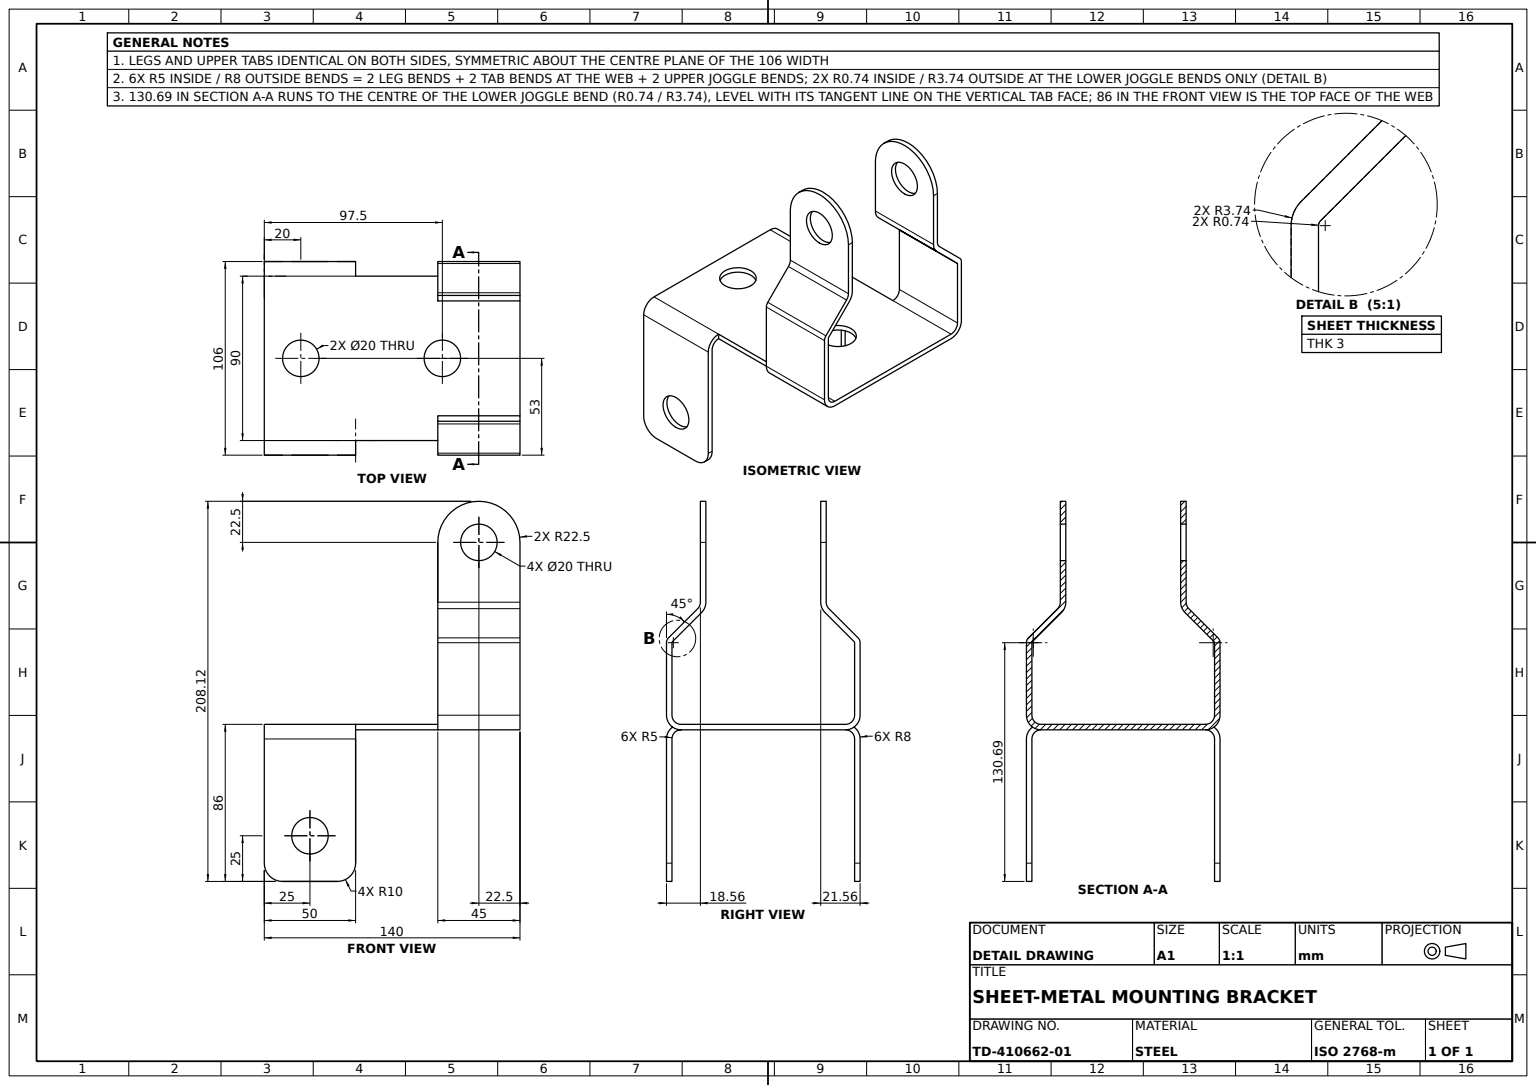
solid
v1 (-53,-76,70)
v2 (-50,-76,70)
e1 v1 v2 LINE
v3 (-50,-8,70)
e2 v2 v3 LINE
v4 (-53,-8,70)
e3 v3 v4 LINE
e4 v1 v4 LINE
face PLANE(AX(P(-53,-3,70),D(0,0,-1),D(-1,0,0))) rev [e1 e2 e3 -e4]
v5 (0,0,-17.5)
v6 (0,0,-37.5)
e5 v5 v6 CIRCLE(AX(P(0,0,-27.5),D(0,1,0),D(0,0,1)),10)
e6 v6 v5 CIRCLE(AX(P(0,0,-27.5),D(0,1,0),D(0,0,1)),10)
v7 (0,0,60)
v8 (0,0,40)
e7 v7 v8 CIRCLE(AX(P(0,0,50),D(0,1,0),D(0,0,1)),10)
e8 v8 v7 CIRCLE(AX(P(0,0,50),D(0,1,0),D(0,0,1)),10)
v9 (-45,0,-70)
v10 (-45,0,-25)
e9 v9 v10 LINE
v11 (-45,0,20)
e10 v10 v11 LINE
v12 (-45,0,70)
e11 v11 v12 LINE
v13 (45,0,70)
e12 v12 v13 LINE
v14 (45,0,20)
e13 v13 v14 LINE
v15 (45,0,-25)
e14 v14 v15 LINE
v16 (45,0,-70)
e15 v16 v15 LINE
e16 v16 v9 LINE
face PLANE(AX(P(0,0,0),D(0,-1,0),D(0,0,-1))) rev [-e5 -e6] [-e7 -e8] [e9 e10 e11 e12 e13 e14 -e15 e16]
v17 (31.443651,99.61899,-70)
v18 (31.443651,66.870058,-70)
e17 v17 v18 LINE
v19 (34.443651,99.61899,-70)
e18 v17 v19 LINE
v20 (34.443651,66.870058,-70)
e19 v19 v20 LINE
e20 v20 v18 LINE
face PLANE(AX(P(31.443651,64.79899,-70),D(0,0,1),D(1,0,0))) rev [-e17 e18 e19 e20]
v21 (50,5,-25)
e21 v15 v21 CIRCLE(AX(P(45,5,-25),D(0,0,1),D(0,1,0)),5)
v22 (50,5,-70)
e22 v21 v22 LINE
e23 v22 v16 CIRCLE(AX(P(45,5,-70),D(0,0,-1),D(0,1,0)),5)
face CYL(AX(P(45,5,-70),D(0,0,-1),D(1,0,0)),5) rev [e21 e22 e23 e15]
v23 (50,44.69489,-70)
v24 (53,44.69489,-70)
e24 v23 v24 LINE
v25 (49.784255,45.215745,-70)
e25 v25 v23 CIRCLE(AX(P(49.2634,44.69489,-70),D(0,0,-1),D(-1,0,0)),0.7366)
v26 (51.905575,47.337065,-70)
e26 v25 v26 LINE
e27 v26 v24 CIRCLE(AX(P(49.2634,44.69489,-70),D(0,0,-1),D(-1,0,0)),3.7366)
face PLANE(AX(P(49.2634,44.69489,-70),D(0,0,1),D(1,0,0))) rev [-e24 -e25 e26 e27]
v27 (-53,44.69489,-70)
v28 (-51.905575,47.337065,-70)
e28 v27 v28 CIRCLE(AX(P(-49.2634,44.69489,-70),D(0,0,-1),D(1,0,0)),3.7366)
v29 (-49.784255,45.215745,-70)
e29 v29 v28 LINE
v30 (-50,44.69489,-70)
e30 v30 v29 CIRCLE(AX(P(-49.2634,44.69489,-70),D(0,0,-1),D(1,0,0)),0.7366)
e31 v30 v27 LINE
face PLANE(AX(P(-49.2634,44.69489,-70),D(0,0,-1),D(-1,0,0))) [e28 -e29 -e30 e31]
v31 (-53,-8,20)
e32 v31 v4 LINE
v32 (-53,-76,20)
e33 v31 v32 LINE
v33 (-53,-86,30)
e34 v32 v33 CIRCLE(AX(P(-53,-76,30),D(-1,0,0),D(0,1,0)),10)
v34 (-53,-86,60)
e35 v33 v34 LINE
e36 v34 v1 CIRCLE(AX(P(-53,-76,60),D(-1,0,0),D(0,1,0)),10)
v35 (-53,-71,45)
v36 (-53,-51,45)
e37 v35 v36 CIRCLE(AX(P(-53,-61,45),D(-1,0,0),D(0,-1,0)),10)
e38 v36 v35 CIRCLE(AX(P(-53,-61,45),D(-1,0,0),D(0,-1,0)),10)
face PLANE(AX(P(-53,0,0),D(1,0,0),D(0,1,0))) rev [-e32 e33 e34 e35 e36 e4] [-e37 -e38]
v37 (-34.443651,66.870058,-25)
v38 (-31.443651,66.870058,-25)
e39 v37 v38 LINE
v39 (-35.908117,63.334524,-25)
e40 v39 v37 CIRCLE(AX(P(-39.443651,66.870058,-25),D(0,0,1),D(-1,0,0)),5)
v40 (-33.786797,61.213203,-25)
e41 v39 v40 LINE
e42 v40 v38 CIRCLE(AX(P(-39.443651,66.870058,-25),D(0,0,1),D(-1,0,0)),8)
face PLANE(AX(P(-39.443651,66.870058,-25),D(0,0,1),D(1,0,0))) [-e39 -e40 e41 e42]
v41 (-51.905575,47.337065,-25)
v42 (-53,44.69489,-25)
e43 v41 v42 CIRCLE(AX(P(-49.2634,44.69489,-25),D(0,0,1),D(1,0,0)),3.7366)
v43 (-50,44.69489,-25)
e44 v43 v42 LINE
v44 (-49.784255,45.215745,-25)
e45 v44 v43 CIRCLE(AX(P(-49.2634,44.69489,-25),D(0,0,1),D(1,0,0)),0.7366)
e46 v44 v41 LINE
face PLANE(AX(P(-49.2634,44.69489,-25),D(0,0,-1),D(-1,0,0))) rev [e43 -e44 -e45 e46]
v45 (53,-76,70)
v46 (53,-86,60)
e47 v45 v46 CIRCLE(AX(P(53,-76,60),D(1,0,0),D(0,-1,0)),10)
v47 (50,-76,70)
e48 v47 v45 LINE
v48 (50,-86,60)
e49 v48 v47 CIRCLE(AX(P(50,-76,60),D(-1,0,0),D(0,-1,0)),10)
e50 v46 v48 LINE
face CYL(AX(P(53,-76,60),D(-1,0,0),D(0,-1,0)),10) [-e47 -e48 -e49 -e50]
v49 (45,-3,20)
e51 v49 v14 LINE
v50 (53,-8,20)
e52 v14 v50 CIRCLE(AX(P(45,-8,20),D(0,0,-1),D(0,-1,0)),8)
v51 (50,-8,20)
e53 v51 v50 LINE
e54 v49 v51 CIRCLE(AX(P(45,-8,20),D(0,0,-1),D(0,-1,0)),5)
face PLANE(AX(P(45,-8,20),D(0,0,-1),D(0,1,0))) [e51 e52 -e53 -e54]
v52 (0,-3,-37.5)
v53 (0,-3,-17.5)
e55 v52 v53 CIRCLE(AX(P(0,-3,-27.5),D(0,-1,0),D(0,0,-1)),10)
e56 v53 v5 LINE
e57 v52 v6 LINE
face CYL(AX(P(0,-10,-27.5),D(0,1,0),D(0,0,1)),10) rev [e55 e56 e5 -e57]
v54 (-45,-3,-70)
v55 (-53,5,-70)
e58 v54 v55 CIRCLE(AX(P(-45,5,-70),D(0,0,-1),D(0,-1,0)),8)
v56 (-50,5,-70)
e59 v56 v55 LINE
e60 v9 v56 CIRCLE(AX(P(-45,5,-70),D(0,0,-1),D(0,-1,0)),5)
e61 v54 v9 LINE
face PLANE(AX(P(-45,5,-70),D(0,0,-1),D(0,1,0))) [e58 -e59 -e60 -e61]
e62 v53 v52 CIRCLE(AX(P(0,-3,-27.5),D(0,-1,0),D(0,0,-1)),10)
face CYL(AX(P(0,-10,-27.5),D(0,1,0),D(0,0,1)),10) rev [e62 e57 e6 -e56]
v57 (50,44.69489,-25)
v58 (53,44.69489,-25)
e63 v57 v58 LINE
e64 v57 v21 LINE
v59 (53,5,-25)
e65 v21 v59 LINE
e66 v58 v59 LINE
face PLANE(AX(P(53,0,-25),D(0,0,-1),D(0,1,0))) rev [-e63 e64 e65 -e66]
v60 (45,-3,70)
e67 v60 v13 LINE
v61 (-45,-3,70)
e68 v61 v12 LINE
e69 v61 v60 LINE
face PLANE(AX(P(-45,-3,70),D(0,0,1),D(1,0,0))) [e67 -e12 -e68 e69]
v62 (-45,-3,-25)
e70 v54 v62 LINE
v63 (-53,5,-25)
e71 v63 v62 CIRCLE(AX(P(-45,5,-25),D(0,0,1),D(0,-1,0)),8)
e72 v63 v55 LINE
face CYL(AX(P(-45,5,-25),D(0,0,1),D(-1,0,0)),8) [-e58 e70 -e71 e72]
v64 (50,-71,45)
v65 (53,-71,45)
e73 v64 v65 LINE
v66 (50,-51,45)
e74 v64 v66 CIRCLE(AX(P(50,-61,45),D(-1,0,0),D(0,-1,0)),10)
v67 (53,-51,45)
e75 v66 v67 LINE
e76 v67 v65 CIRCLE(AX(P(53,-61,45),D(1,0,0),D(0,1,0)),10)
face CYL(AX(P(-45,-61,45),D(1,0,0),D(0,1,0)),10) rev [-e73 e74 e75 e76]
e77 v66 v64 CIRCLE(AX(P(50,-61,45),D(-1,0,0),D(0,-1,0)),10)
v68 (50,-86,30)
e78 v48 v68 LINE
v69 (50,-8,70)
e79 v69 v47 LINE
e80 v51 v69 LINE
v70 (50,-76,20)
e81 v70 v51 LINE
e82 v70 v68 CIRCLE(AX(P(50,-76,30),D(-1,0,0),D(0,-1,0)),10)
face PLANE(AX(P(50,0,0),D(-1,0,0),D(0,-1,0))) [-e77 -e74] [-e78 e49 -e79 -e80 -e81 e82]
v71 (34.443651,66.870058,-25)
v72 (34.443651,99.61899,-25)
e83 v71 v72 LINE
e84 v20 v71 LINE
v73 (34.443651,122.11899,-47.5)
e85 v19 v73 CIRCLE(AX(P(34.443651,99.61899,-47.5),D(1,0,0),D(0,1,0)),22.5)
e86 v73 v72 CIRCLE(AX(P(34.443651,99.61899,-47.5),D(1,0,0),D(0,1,0)),22.5)
v74 (34.443651,109.61899,-47.5)
v75 (34.443651,89.61899,-47.5)
e87 v74 v75 CIRCLE(AX(P(34.443651,99.61899,-47.5),D(1,0,0),D(0,1,0)),10)
e88 v75 v74 CIRCLE(AX(P(34.443651,99.61899,-47.5),D(1,0,0),D(0,1,0)),10)
face PLANE(AX(P(34.443651,0,0),D(1,0,0),D(0,1,0))) [-e83 -e84 -e19 e85 e86] [-e87 -e88]
e89 v31 v11 CIRCLE(AX(P(-45,-8,20),D(0,0,-1),D(0,1,0)),8)
v76 (-45,-3,20)
e90 v76 v11 LINE
v77 (-50,-8,20)
e91 v77 v76 CIRCLE(AX(P(-45,-8,20),D(0,0,-1),D(0,1,0)),5)
e92 v77 v31 LINE
face PLANE(AX(P(-45,-8,20),D(0,0,1),D(0,-1,0))) rev [e89 -e90 -e91 e92]
v78 (35.908117,63.334524,-70)
v79 (33.786797,61.213203,-70)
e93 v78 v79 LINE
e94 v26 v78 LINE
e95 v25 v79 LINE
face PLANE(AX(P(34.443651,64.79899,-70),D(0,0,1),D(1,0,0))) rev [-e93 -e94 -e26 e95]
e96 v76 v61 LINE
e97 v61 v3 CIRCLE(AX(P(-45,-8,70),D(0,0,1),D(0,1,0)),5)
e98 v3 v77 LINE
face CYL(AX(P(-45,-8,20),D(0,0,-1),D(-1,0,0)),5) rev [e96 e97 e98 e91]
v80 (-50,-86,60)
e99 v80 v34 LINE
v81 (-50,-86,30)
e100 v33 v81 LINE
e101 v81 v80 LINE
face PLANE(AX(P(-53,-86,70),D(0,1,0),D(-1,0,0))) rev [e99 -e35 e100 e101]
v82 (31.443651,66.870058,-25)
v83 (31.443651,99.61899,-25)
e102 v82 v83 LINE
e103 v71 v82 LINE
e104 v72 v83 LINE
face PLANE(AX(P(31.443651,122.11899,-25),D(0,0,-1),D(-1,0,0))) rev [-e102 -e103 e83 e104]
e105 v69 v60 CIRCLE(AX(P(45,-8,70),D(0,0,1),D(0,-1,0)),5)
v84 (53,-8,70)
e106 v69 v84 LINE
e107 v84 v13 CIRCLE(AX(P(45,-8,70),D(0,0,1),D(0,-1,0)),8)
face PLANE(AX(P(45,-8,70),D(0,0,-1),D(0,1,0))) rev [-e67 -e105 e106 e107]
v85 (33.786797,61.213203,-25)
e108 v85 v79 LINE
v86 (49.784255,45.215745,-25)
e109 v86 v25 LINE
e110 v85 v86 LINE
face PLANE(AX(P(47.5,47.5,0),D(-0.707106781,-0.707106781,0),D(0.707106781,-0.707106781,0))) [e108 -e95 -e109 -e110]
v87 (53,5,-70)
e111 v22 v87 LINE
v88 (45,-3,-70)
e112 v87 v88 CIRCLE(AX(P(45,5,-70),D(0,0,-1),D(0,1,0)),8)
e113 v88 v16 LINE
face PLANE(AX(P(45,5,-70),D(0,0,1),D(0,-1,0))) rev [-e23 e111 e112 e113]
e114 v43 v30 LINE
e115 v29 v44 LINE
face CYL(AX(P(-49.2634,44.69489,-25),D(0,0,1),D(-0.707106781,0.707106781,0)),0.7366) rev [e114 e30 e115 e45]
v89 (-50,5,-25)
e116 v43 v89 LINE
e117 v56 v89 LINE
e118 v56 v30 LINE
face PLANE(AX(P(-50,0,0),D(1,0,0),D(0,-1,0))) [e116 -e117 e118 -e114]
v90 (-31.443651,66.870058,-70)
e119 v90 v38 LINE
v91 (-33.786797,61.213203,-70)
e120 v91 v40 LINE
e121 v90 v91 CIRCLE(AX(P(-39.443651,66.870058,-70),D(0,0,-1),D(-1,0,0)),8)
face CYL(AX(P(-39.443651,66.870058,-70),D(0,0,-1),D(1,0,0)),8) [e119 -e42 -e120 -e121]
e122 v89 v10 CIRCLE(AX(P(-45,5,-25),D(0,0,1),D(0,-1,0)),5)
e123 v89 v63 LINE
e124 v10 v62 LINE
face PLANE(AX(P(-45,5,-25),D(0,0,-1),D(0,1,0))) rev [-e122 e123 e71 -e124]
e125 v79 v18 CIRCLE(AX(P(39.443651,66.870058,-70),D(0,0,-1),D(1,0,0)),8)
e126 v78 v20 CIRCLE(AX(P(39.443651,66.870058,-70),D(0,0,-1),D(1,0,0)),5)
face PLANE(AX(P(39.443651,66.870058,-70),D(0,0,-1),D(-1,0,0))) [e93 e125 -e20 -e126]
e127 v82 v85 CIRCLE(AX(P(39.443651,66.870058,-25),D(0,0,1),D(1,0,0)),8)
v92 (35.908117,63.334524,-25)
e128 v92 v85 LINE
e129 v71 v92 CIRCLE(AX(P(39.443651,66.870058,-25),D(0,0,1),D(1,0,0)),5)
face PLANE(AX(P(39.443651,66.870058,-25),D(0,0,-1),D(-1,0,0))) rev [e103 e127 -e128 -e129]
v93 (-31.443651,99.61899,-25)
v94 (-34.443651,99.61899,-25)
e130 v93 v94 LINE
v95 (-31.443651,99.61899,-70)
e131 v95 v93 CIRCLE(AX(P(-31.443651,99.61899,-47.5),D(1,0,0),D(0,-1,0)),22.5)
v96 (-34.443651,99.61899,-70)
e132 v96 v95 LINE
e133 v94 v96 CIRCLE(AX(P(-34.443651,99.61899,-47.5),D(-1,0,0),D(0,-1,0)),22.5)
face CYL(AX(P(-31.443651,99.61899,-47.5),D(-1,0,0),D(0,-1,0)),22.5) [-e130 -e131 -e132 -e133]
v97 (51.905575,47.337065,-25)
e134 v26 v97 LINE
e135 v58 v97 CIRCLE(AX(P(49.2634,44.69489,-25),D(0,0,1),D(-1,0,0)),3.7366)
e136 v24 v58 LINE
face CYL(AX(P(49.2634,44.69489,-70),D(0,0,-1),D(0.707106781,0.707106781,0)),3.7366) [e134 -e135 -e136 -e27]
v98 (31.443651,89.61899,-47.5)
e137 v98 v75 LINE
v99 (31.443651,109.61899,-47.5)
e138 v99 v98 CIRCLE(AX(P(31.443651,99.61899,-47.5),D(1,0,0),D(0,1,0)),10)
e139 v99 v74 LINE
face CYL(AX(P(24.443651,99.61899,-47.5),D(1,0,0),D(0,1,0)),10) rev [e87 -e137 -e138 e139]
e140 v87 v59 LINE
e141 v87 v24 LINE
face PLANE(AX(P(53,0,0),D(-1,0,0),D(0,-1,0))) rev [e136 e66 -e140 e141]
e142 v88 v54 LINE
face PLANE(AX(P(-45,-3,-70),D(0,0,-1),D(-1,0,0))) [e61 -e16 -e113 e142]
v100 (-50,-71,45)
e143 v100 v35 LINE
v101 (-50,-51,45)
e144 v100 v101 CIRCLE(AX(P(-50,-61,45),D(1,0,0),D(0,1,0)),10)
e145 v101 v36 LINE
face CYL(AX(P(-43,-61,45),D(-1,0,0),D(0,-1,0)),10) rev [e38 -e143 e144 e145]
v102 (-31.443651,89.61899,-47.5)
v103 (-31.443651,109.61899,-47.5)
e146 v102 v103 CIRCLE(AX(P(-31.443651,99.61899,-47.5),D(1,0,0),D(0,-1,0)),10)
e147 v103 v102 CIRCLE(AX(P(-31.443651,99.61899,-47.5),D(1,0,0),D(0,-1,0)),10)
e148 v95 v90 LINE
e149 v38 v93 LINE
face PLANE(AX(P(-31.443651,0,0),D(-1,0,0),D(0,1,0))) rev [-e146 -e147] [-e148 e131 -e149 -e119]
e150 v92 v78 LINE
e151 v92 v97 LINE
face PLANE(AX(P(49.62132,49.62132,0),D(-0.707106781,-0.707106781,0),D(0.707106781,-0.707106781,0))) rev [-e134 e94 -e150 e151]
v104 (45,-3,-25)
e152 v104 v59 CIRCLE(AX(P(45,5,-25),D(0,0,1),D(0,1,0)),8)
e153 v88 v104 LINE
face CYL(AX(P(45,5,-70),D(0,0,-1),D(1,0,0)),8) [e140 -e152 -e153 -e112]
v105 (-50,-76,20)
e154 v105 v32 LINE
e155 v81 v105 CIRCLE(AX(P(-50,-76,30),D(1,0,0),D(0,1,0)),10)
face CYL(AX(P(-53,-76,30),D(1,0,0),D(0,1,0)),10) [-e154 -e155 -e100 -e34]
v106 (53,-86,30)
e156 v46 v106 LINE
e157 v68 v106 LINE
face PLANE(AX(P(53,-86,20),D(0,1,0),D(-1,0,0))) rev [-e156 e50 e78 e157]
e158 v60 v49 LINE
e159 v62 v76 LINE
e160 v49 v104 LINE
v107 (0,-3,60)
v108 (0,-3,40)
e161 v107 v108 CIRCLE(AX(P(0,-3,50),D(0,-1,0),D(0,0,-1)),10)
e162 v108 v107 CIRCLE(AX(P(0,-3,50),D(0,-1,0),D(0,0,-1)),10)
face PLANE(AX(P(0,-3,0),D(0,-1,0),D(0,0,-1))) [-e158 -e69 -e96 -e159 -e70 -e142 e153 -e160] [-e62 -e55] [-e161 -e162]
e163 v15 v104 LINE
face PLANE(AX(P(45,5,-25),D(0,0,1),D(0,-1,0))) [-e65 -e21 e163 e152]
v109 (-34.443651,66.870058,-70)
e164 v96 v109 LINE
e165 v109 v90 LINE
face PLANE(AX(P(-31.443651,64.79899,-70),D(0,0,-1),D(-1,0,0))) [-e164 e132 e148 -e165]
e166 v86 v97 LINE
face PLANE(AX(P(52.12132,47.12132,-25),D(0,0,-1),D(0,1,0))) rev [e166 -e151 e128 e110]
e167 v84 v50 LINE
face CYL(AX(P(45,-8,70),D(0,0,1),D(1,0,0)),8) [e167 -e52 -e13 -e107]
e168 v77 v105 LINE
face PLANE(AX(P(-53,-86,20),D(0,0,1),D(0,-1,0))) rev [e154 -e33 -e92 e168]
v110 (-35.908117,63.334524,-70)
e169 v110 v39 LINE
e170 v37 v109 LINE
e171 v109 v110 CIRCLE(AX(P(-39.443651,66.870058,-70),D(0,0,-1),D(-1,0,0)),5)
face CYL(AX(P(-39.443651,66.870058,-70),D(0,0,-1),D(1,0,0)),5) rev [e169 e40 e170 e171]
face CYL(AX(P(-45,5,-25),D(0,0,1),D(-1,0,0)),5) rev [e122 -e9 e60 e117]
e172 v42 v63 LINE
face PLANE(AX(P(-53,0,-25),D(0,0,1),D(0,-1,0))) [e172 -e123 -e116 e44]
v111 (-34.443651,89.61899,-47.5)
e173 v102 v111 LINE
v112 (-34.443651,109.61899,-47.5)
e174 v103 v112 LINE
e175 v111 v112 CIRCLE(AX(P(-34.443651,99.61899,-47.5),D(1,0,0),D(0,1,0)),10)
face CYL(AX(P(-24.443651,99.61899,-47.5),D(-1,0,0),D(0,-1,0)),10) rev [-e173 e146 e174 -e175]
e176 v12 v4 CIRCLE(AX(P(-45,-8,70),D(0,0,1),D(0,1,0)),8)
face CYL(AX(P(-45,-8,20),D(0,0,-1),D(-1,0,0)),8) [-e11 -e89 e32 -e176]
e177 v101 v100 CIRCLE(AX(P(-50,-61,45),D(1,0,0),D(0,1,0)),10)
e178 v2 v80 CIRCLE(AX(P(-50,-76,60),D(1,0,0),D(0,1,0)),10)
face PLANE(AX(P(-50,0,0),D(1,0,0),D(0,1,0))) [-e144 -e177] [e155 -e168 -e98 -e2 e178 -e101]
e179 v55 v27 LINE
face PLANE(AX(P(-53,45,-70),D(0,0,-1),D(-1,0,0))) [-e31 -e118 e59 e179]
e180 v98 v99 CIRCLE(AX(P(31.443651,99.61899,-47.5),D(1,0,0),D(0,1,0)),10)
face CYL(AX(P(24.443651,99.61899,-47.5),D(1,0,0),D(0,1,0)),10) rev [-e139 -e180 e137 e88]
e181 v57 v86 CIRCLE(AX(P(49.2634,44.69489,-25),D(0,0,1),D(-1,0,0)),0.7366)
face PLANE(AX(P(49.2634,44.69489,-25),D(0,0,1),D(1,0,0))) [e135 -e166 -e181 e63]
e182 v65 v67 CIRCLE(AX(P(53,-61,45),D(1,0,0),D(0,1,0)),10)
v113 (53,-76,20)
e183 v106 v113 CIRCLE(AX(P(53,-76,30),D(1,0,0),D(0,-1,0)),10)
e184 v113 v50 LINE
e185 v84 v45 LINE
face PLANE(AX(P(53,0,0),D(-1,0,0),D(0,-1,0))) rev [-e76 -e182] [e156 e183 e184 -e167 e185 e47]
e186 v41 v28 LINE
e187 v42 v27 LINE
face CYL(AX(P(-49.2634,44.69489,-25),D(0,0,1),D(-0.707106781,0.707106781,0)),3.7366) [-e43 e186 -e28 -e187]
face CYL(AX(P(45,-8,70),D(0,0,1),D(1,0,0)),5) rev [e105 e158 e54 e80]
face PLANE(AX(P(45,-3,70),D(1,0,0),D(0,0,-1))) [-e51 e160 -e163 -e14]
e188 v110 v91 LINE
e189 v29 v91 LINE
e190 v28 v110 LINE
face PLANE(AX(P(-34.443651,64.79899,-70),D(0,0,-1),D(-1,0,0))) [e188 -e189 e29 e190]
v114 (31.443651,122.11899,-47.5)
e191 v83 v114 CIRCLE(AX(P(31.443651,99.61899,-47.5),D(-1,0,0),D(0,1,0)),22.5)
e192 v114 v73 LINE
face CYL(AX(P(34.443651,99.61899,-47.5),D(1,0,0),D(0,1,0)),22.5) [-e191 -e104 -e86 -e192]
face CYL(AX(P(-53,-76,60),D(1,0,0),D(0,1,0)),10) [-e36 -e99 -e178 -e1]
face PLANE(AX(P(-45,-8,70),D(0,0,1),D(0,-1,0))) [e176 -e3 -e97 e68]
e193 v114 v17 CIRCLE(AX(P(31.443651,99.61899,-47.5),D(-1,0,0),D(0,1,0)),22.5)
e194 v82 v18 LINE
face PLANE(AX(P(31.443651,0,0),D(1,0,0),D(0,1,0))) rev [e102 e191 e193 e17 -e194] [e180 e138]
face CYL(AX(P(39.443651,66.870058,-25),D(0,0,1),D(-1,0,0)),5) rev [e129 e150 e126 e84]
e195 v40 v44 LINE
face PLANE(AX(P(-47.5,47.5,0),D(0.707106781,-0.707106781,0),D(-0.707106781,-0.707106781,0))) [-e115 e189 e120 e195]
face PLANE(AX(P(53,-86,70),D(0,0,-1),D(-1,0,0))) rev [e79 e48 -e185 -e106]
e196 v107 v7 LINE
e197 v108 v8 LINE
face CYL(AX(P(0,-10,50),D(0,1,0),D(0,0,1)),10) rev [e162 e196 e7 -e197]
e198 v37 v94 LINE
face PLANE(AX(P(-31.443651,122.11899,-25),D(0,0,1),D(1,0,0))) [e149 e130 -e198 e39]
face PLANE(AX(P(-45,-3,70),D(-1,0,0),D(0,0,1))) [e159 e90 -e10 e124]
e199 v22 v23 LINE
face PLANE(AX(P(53,45,-70),D(0,0,1),D(1,0,0))) rev [-e111 e199 e24 -e141]
e200 v23 v57 LINE
face CYL(AX(P(49.2634,44.69489,-70),D(0,0,-1),D(0.707106781,0.707106781,0)),0.7366) rev [e181 e109 e25 e200]
e201 v112 v111 CIRCLE(AX(P(-34.443651,99.61899,-47.5),D(1,0,0),D(0,1,0)),10)
face PLANE(AX(P(-34.443651,0,0),D(-1,0,0),D(0,1,0))) [e175 e201] [e198 e133 e164 -e170]
e202 v113 v70 LINE
face CYL(AX(P(53,-76,30),D(-1,0,0),D(0,-1,0)),10) [-e202 -e183 -e157 -e82]
face CYL(AX(P(-45,-61,45),D(1,0,0),D(0,1,0)),10) rev [e77 e73 e182 -e75]
face PLANE(AX(P(50,0,0),D(-1,0,0),D(0,-1,0))) [-e199 -e22 -e64 -e200]
face PLANE(AX(P(-53,0,0),D(1,0,0),D(0,-1,0))) rev [-e172 e187 -e179 -e72]
face PLANE(AX(P(53,-3,20),D(0,0,1),D(1,0,0))) rev [e81 e53 -e184 e202]
face CYL(AX(P(-24.443651,99.61899,-47.5),D(-1,0,0),D(0,-1,0)),10) rev [e147 e173 -e201 -e174]
e203 v39 v41 LINE
face PLANE(AX(P(-52.12132,47.12132,-25),D(0,0,1),D(0,-1,0))) [-e46 -e195 -e41 e203]
face CYL(AX(P(0,-10,50),D(0,1,0),D(0,0,1)),10) rev [e8 -e196 e161 e197]
face CYL(AX(P(-43,-61,45),D(-1,0,0),D(0,-1,0)),10) rev [e177 e143 e37 -e145]
face PLANE(AX(P(-39.443651,66.870058,-70),D(0,0,1),D(1,0,0))) rev [e165 e121 -e188 -e171]
face CYL(AX(P(34.443651,99.61899,-47.5),D(1,0,0),D(0,1,0)),22.5) [-e18 -e193 e192 -e85]
face CYL(AX(P(39.443651,66.870058,-25),D(0,0,1),D(-1,0,0)),8) [e194 -e125 -e108 -e127]
face PLANE(AX(P(-49.62132,49.62132,0),D(0.707106781,-0.707106781,0),D(-0.707106781,-0.707106781,0))) rev [-e169 -e190 -e186 -e203]
